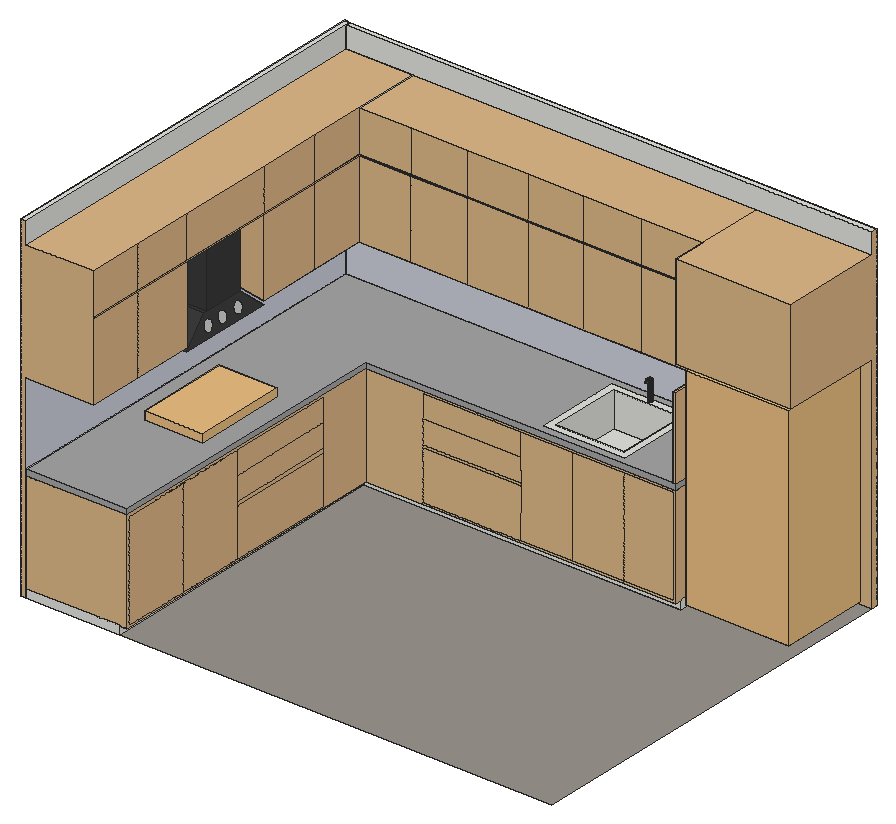
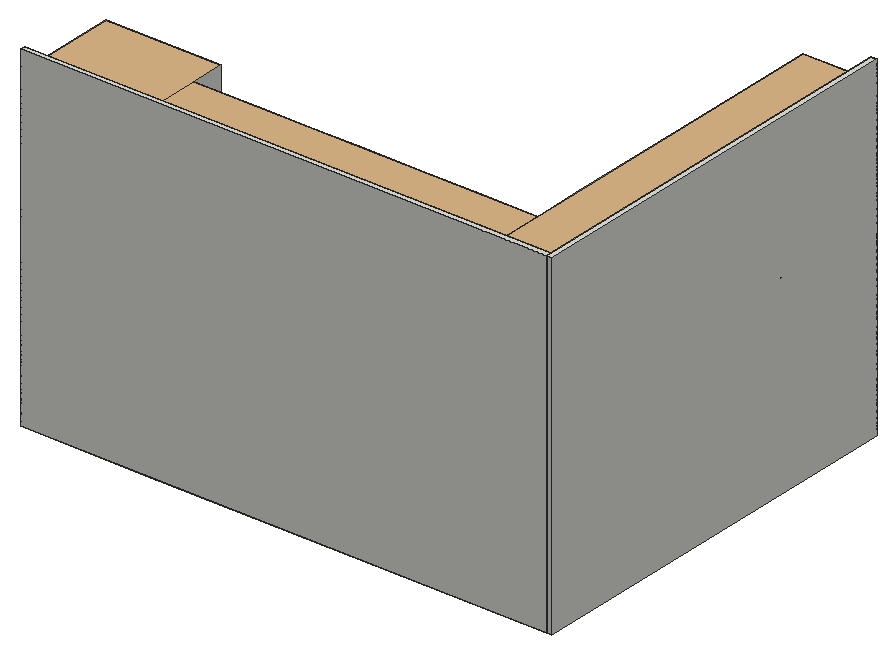
# SketchUp Ruby script. Lengths in inches.
U = 1.inch
M = Sketchup.active_model
def pt(a) = Geom::Point3d.new(a.map { |v| v * U })
def face(e, loops, mat)
  f = e.add_face(loops[0].map { |a| pt(a) })
  loops[1..].each { |l| e.add_face(l.map { |a| pt(a) }).erase! }
  f.material = f.back_material = mat if mat
  f
end
# faces: each face lists its corners as indices into pts; further lists are holes
def faces(e, pts, list, mat = nil) = list.each { |f| face(e, (f[0].is_a?(Array) ? f : [f]).map { |l| l.map { |i| pts[i] } }, mat) }
# xy, xz, yz: faces in a plane at the given z, y or x. An outline is a flat list of corners, or four numbers for a rectangle; further outlines are holes
def ring(l) = l.size == 4 ? [[l[0], l[1]], [l[2], l[1]], [l[2], l[3]], [l[0], l[3]]] : l.each_slice(2).to_a
def flat(e, list, mat, &to3) = list.each { |f| face(e, (f[0].is_a?(Array) ? f : [f]).map { |l| ring(l).map { |u, v| to3.(u, v) } }, mat) }
def xy(e, z, list, mat = nil) = flat(e, list, mat) { |x, y| [x, y, z] }
def xz(e, y, list, mat = nil) = flat(e, list, mat) { |x, z| [x, y, z] }
def yz(e, x, list, mat = nil) = flat(e, list, mat) { |y, z| [x, y, z] }
def lines(e, pts, list) = list.each { |a, b| e.add_line(pt(pts[a]), pt(pts[b])) }
# prism: a flat outline (further loops are holes) pulled along v
def prism(e, loops, v, mat = nil)
  f = face(e, loops, mat); d = Geom::Vector3d.new(v.map { |x| x * U })
  f.pushpull(f.normal.samedirection?(d) ? d.length : -d.length)
end
def box(e, o, s, mat = nil) = prism(e, [[o, [o[0] + s[0], o[1], o[2]], [o[0] + s[0], o[1] + s[1], o[2]], [o[0], o[1] + s[1], o[2]]]], [0, 0, s[2]], mat)
def at(x, y, z, deg = 0) = Geom::Transformation.translation(pt([x, y, z])) * Geom::Transformation.rotation(ORIGIN, Z_AXIS, deg.degrees)
def axes(o, x, y, z) = Geom::Transformation.new([*x, 0, *y, 0, *z, 0, *pt(o).to_a, 1])
def part(name) = M.definitions.add(name)
# library, detail: a bought-in or finely detailed component or shape, given as its bounding box
def library(name, o, s) = part(name).tap { |d| box(d.entities, o, s) }
def detail(e, o, s) = box(e.add_group.entities, o, s)
def put(e, d, t, mat = nil) = e.add_instance(d, t).tap { |i| i.material = mat if mat }
def group(e, t, mat = nil) = e.add_group.tap { |g| g.transformation = t; g.material = mat if mat }.entities
root = M.entities
M.materials.add("[0036_BurlyWood]").color = [222, 184, 135]
M.materials.add("[Color M02]").color = [198, 198, 198]
M.materials.add("[Color M06]").color = [86, 86, 86]
M.materials.add("[Color M07]").color = [58, 58, 58]
M.materials.add("[Granite Tile]").color = [155, 148, 143]
M.materials.add("[Marble Carrara Floor Tile]").color = [204, 208, 219]
M.materials.add("[Stone Vein Gray]").color = [166, 165, 165]
c1 = library("Group\#3",[0,0,0],[36.5,31.625,66.0625])
xy(root,0,[[0,0,2,144],[2,0,2,142,147.9375,142,147.9375,108.5,35.1875,108.5,35.1875,0],[2,142,147.9375,144],[147.9375,142,188.9375,144]])
xy(root,0,[[35.1875,0,35.1875,108.5,147.9375,108.5,147.9375,142,188.9375,142,188.9375,0]],"[Granite Tile]")
xy(root,3,[[2,0,2,142,147.9375,142,147.9375,108.5,35.1875,108.5,35.1875,0],[35.1875,0,38,108.5],[38,106,147.9375,108.5]])
xy(root,28,[[3.713,1.713,36.287,1.713,36.287,107.713,146.224,107.713,146.224,140.287,3.713,140.287]])
xy(root,28.6875,[[101.152,111.388,125.325,136.999]])
xy(root,39,[[[2,0,2,142,147.9375,142,147.9375,106,38,106,38,0],[3.713,1.713,36.287,1.713,36.287,107.713,146.224,107.713,146.224,140.287,3.713,140.287]]])
xy(root,41,[[[98.739,108.975,127.739,139.412],[101.152,111.388,125.325,136.999],[113.239,137.739,113.065,137.762,112.904,137.829,112.765,137.935,112.658,138.074,112.591,138.236,112.569,138.409,112.591,138.582,112.658,138.744,112.765,138.883,112.904,138.989,113.065,139.056,113.239,139.079,113.412,139.056,113.573,138.989,113.712,138.883,113.819,138.744,113.886,138.582,113.908,138.409,113.886,138.236,113.819,138.074,113.712,137.935,113.573,137.829,113.412,137.762]],[113.239,137.739,113.065,137.762,112.904,137.829,112.765,137.935,112.658,138.074,112.591,138.236,112.569,138.409,112.591,138.582,112.658,138.744,112.765,138.883,112.904,138.989,113.065,139.056,113.239,139.079,113.412,139.056,113.573,138.989,113.712,138.883,113.819,138.744,113.886,138.582,113.908,138.409,113.886,138.236,113.819,138.074,113.712,137.935,113.573,137.829,113.412,137.762]])
xy(root,41,[[146.9375,106,147.9375,142]],"[0036_BurlyWood]")
xy(root,41,[[[2,0,38,0,38,106,146.9375,106,146.9375,142,2,142],[98.739,108.975,127.739,139.412]]],"[Stone Vein Gray]")
xy(root,70,[[2,0,26,41.497],[26,75.622,2,79.962,2,142,26,142],[146.9375,106,147.9375,118],[26,118,146.9375,142],[146.9375,118,147.9375,142]],"[0036_BurlyWood]")
xy(root,79.249,[[147.9375,106,188.9375,142]],"[0036_BurlyWood]")
xy(root,97.4375,[[2,41.497,2,79.962,26,75.622,26,41.497]])
xy(root,97.613,[[125.9375,117.875,147.9375,118]],"[0036_BurlyWood]")
xy(root,97.614,[[26,0,26.3125,118],[26.3125,117.875,44.25,118],[44.25,117.875,64.75,118],[64.75,117.875,86,118],[86,117.875,105.3125,118],
  [105.3125,117.875,125.9375,118]],"[0036_BurlyWood]")
xy(root,97.929,[[26,0,26.3125,118],[26.3125,117.875,44.25,118],[44.25,117.875,64.75,118],[64.75,117.875,86,118],[86,117.875,105.3125,118],
  [105.3125,117.875,147.9375,118]],"[0036_BurlyWood]")
xy(root,112.601,[[2,0,26,142],[147.9375,106,188.9375,142],[26,118,147.9375,142]],"[0036_BurlyWood]")
xy(root,120,[[0,0,2,144],[2,142,188.9375,144]])
xz(root,0,[[2,0,35.1875,3]])
xz(root,0,[[0,0,2,0,2,70,26,70,26,97.614,26.3125,97.614,26.3125,97.929,26,97.929,26,112.601,2,112.601,2,120,0,120],[2,3,38,39]],"[0036_BurlyWood]")
xz(root,0,[[2,39,38,41]],"[Stone Vein Gray]")
xz(root,1.713,[[3.713,28,36.287,39]])
xz(root,41.497,[[2,70,26,97.4375]],"[0036_BurlyWood]")
xz(root,106,[[[38,3,147.9375,39],[58.162,3.56,58.287,21,58.287,21.974,58.224,30.207,58.162,38.44,147.378,38.44,147.378,3.56]],[58.162,3.56,92.787,3.56,92.912,21,58.287,21],[92.787,3.56,111.037,3.56,111.037,38.44,92.787,38.44,92.849,30.207,92.912,21.974,92.912,21],[111.037,3.56,129.537,38.44],[129.537,3.56,147.378,38.44],
  [58.287,21,92.912,21.974],[58.287,21.974,92.912,21.974,92.849,30.207,58.224,30.207],[58.224,30.207,92.849,30.207,92.787,38.44,58.162,38.44],[146.9375,41,147.9375,70],[147.9375,79.249,188.9375,112.601]],"[0036_BurlyWood]")
xz(root,106,[[38,39,147.9375,41]],"[Stone Vein Gray]")
xz(root,107.713,[[36.287,28,146.224,39]])
xz(root,108.5,[[35.1875,0,147.9375,3]])
xz(root,111.388,[[101.152,28.6875,125.325,41]])
xz(root,117.875,[[125.9375,97.613,147.9375,97.613,147.9375,97.929,105.3125,97.929,105.3125,97.614,125.9375,97.614],[26.3125,97.614,44.25,97.929],[44.25,97.614,64.75,97.929],[64.75,97.614,86,97.929],[86,97.614,105.3125,97.929]],"[0036_BurlyWood]")
xz(root,118,[[26,97.614,26.3125,97.8],[26,97.8,26.3125,97.929]])
xz(root,118,[[26,70,44.25,97.614],[44.25,70,64.75,97.614],[64.75,70,86,97.614],[86,70,105.3125,97.614],[105.3125,70,125.9375,97.614],
  [125.9375,70,147.9375,97.613],[26,97.929,44.25,112.601],[44.25,97.929,64.75,112.601],[64.75,97.929,86,112.601],[86,97.929,105.3125,112.601],
  [105.3125,97.929,125.9375,112.601],[125.9375,97.929,147.9375,112.601]],"[0036_BurlyWood]")
xz(root,136.999,[[101.152,28.6875,125.325,41]])
xz(root,140.287,[[3.713,28,146.224,39]])
xz(root,142,[[2,0,147.9375,3],[2,3,147.9375,39],[2,39,147.9375,41],[2,70,26,112.601],[2,112.601,188.9375,120]])
xz(root,142,[[147.9375,0,188.9375,79.249],[146.9375,41,147.9375,70]],"[0036_BurlyWood]")
xz(root,142,[[2,41,146.9375,70]],"[Marble Carrara Floor Tile]")
xz(root,144,[[0,0,2,120],[2,0,188.9375,120]])
yz(root,0,[[0,0,144,120]])
yz(root,2,[[0,0,142,3],[142,0,144,120],[0,3,142,39],[0,39,142,41],[0,112.601,142,120]])
yz(root,2,[[0,41,142,41,142,70,79.962,70,79.962,97.4375,41.497,97.4375,41.497,70,0,70]],"[Marble Carrara Floor Tile]")
yz(root,3.713,[[1.713,28,140.287,39]])
yz(root,26,[[118,70,142,112.601],[41.497,97.4375,75.622,97.614]])
yz(root,26,[[0,70,19.625,97.614],[19.625,70,41.497,97.614],[75.622,70,98.247,97.614],[98.247,70,118,97.614],[0,97.929,19.625,112.601],
  [19.625,97.929,41.497,112.601],[41.497,97.929,75.622,112.601],[75.622,97.929,98.247,112.601],[98.247,97.929,118,112.601]],"[0036_BurlyWood]")
yz(root,26.3125,[[117.875,97.614,118,97.929]])
yz(root,26.3125,[[0,97.614,117.875,97.929]],"[0036_BurlyWood]")
yz(root,35.1875,[[0,0,108.5,3]])
yz(root,36.287,[[1.713,28,107.713,39]])
yz(root,38,[[[0,3,106,39],[0.581,3.581,0.581,38.419,86.83,38.419,86.865,30.341,86.901,21.937,86.901,20.438,86.83,3.581]],[0.581,3.581,24.517,38.419],[24.517,3.581,48.892,3.581,48.963,20.438,48.963,21.937,48.928,30.178,48.892,38.419,24.517,38.419],[48.892,3.581,86.83,3.581,86.901,20.438,48.963,20.438],[48.963,20.438,86.901,21.937],
  [48.963,21.937,86.901,21.937,86.865,30.341,48.928,30.178],[48.928,30.178,86.865,30.341,86.83,38.419,48.892,38.419]],"[0036_BurlyWood]")
yz(root,38,[[0,39,106,41]],"[Stone Vein Gray]")
yz(root,101.152,[[111.388,28.6875,136.999,41]])
yz(root,125.325,[[111.388,28.6875,136.999,38.375],[111.388,38.375,136.999,41]])
yz(root,125.9375,[[117.875,97.613,118,97.614]])
yz(root,146.224,[[107.713,28,140.287,39]])
yz(root,146.9375,[[106,41,142,70]],"[0036_BurlyWood]")
yz(root,147.9375,[[108.5,0,142,3],[106,79.249,106,112.601,118,112.601,118,97.929,117.875,97.929,117.875,97.613,118,97.613,118,79.249]])
yz(root,147.9375,[[106,3,142,39],[106,41,142,70],[118,70,142,79.249]],"[0036_BurlyWood]")
yz(root,147.9375,[[106,39,142,41]],"[Stone Vein Gray]")
yz(root,188.9375,[[142,0,144,0,144,120,142,120,142,112.601,106,112.601,106,79.249,142,79.249]],"[0036_BurlyWood]")
p = [[113.065,137.762,41],[113.239,137.739,41],[113.239,137.739,47.367],[113.239,137.739,47.377],[113.065,137.762,47.381],[113.065,137.762,47.373],
  [113.412,137.762,41],[113.412,137.762,47.373],[113.412,137.762,47.381],[112.765,137.935,41],[112.904,137.829,41],[112.904,137.829,47.394],
  [112.901,137.83,47.394],[112.765,137.935,47.413],[113.573,137.829,41],[113.573,137.829,47.394],[113.712,137.935,41],[113.712,137.935,47.413],
  [113.576,137.83,47.394],[112.658,138.074,41],[112.658,138.074,47.439],[113.819,138.074,41],[113.819,138.074,47.439],[112.591,138.236,41],
  [112.591,138.236,47.468],[113.886,138.236,41],[113.886,138.236,47.468],[112.569,138.409,41],[112.569,138.409,47.5],[113.908,138.409,41],
  [113.908,138.409,47.5],[112.591,138.582,41],[112.591,138.582,47.532],[113.886,138.582,41],[113.886,138.582,47.532],[112.658,138.744,41],
  [112.658,138.744,47.561],[113.819,138.744,41],[113.819,138.744,47.561],[112.765,138.883,41],[112.765,138.883,47.587],[113.712,138.883,41],
  [113.712,138.883,47.587],[112.904,138.989,41],[112.904,138.989,47.606],[113.573,138.989,41],[113.573,138.989,47.606],[113.065,139.056,41],
  [113.065,139.056,47.619],[113.412,139.056,41],[113.412,139.056,47.619],[113.239,139.079,41],[113.239,139.079,47.623],[112.569,136.909,47.5],
  [112.591,137.071,47.439],[112.658,137.222,47.381],[112.765,137.352,47.332],[112.904,137.451,47.294],[113.065,137.514,47.271],[113.239,137.535,47.262],
  [113.412,137.514,47.271],[113.573,137.451,47.294],[113.712,137.352,47.332],[113.819,137.222,47.381],[113.886,137.071,47.439],[113.908,136.909,47.5],
  [113.886,136.747,47.561],[113.819,136.596,47.619],[113.712,136.466,47.668],[113.573,136.366,47.706],[113.412,136.304,47.729],[113.239,136.283,47.738],
  [113.065,136.304,47.729],[112.904,136.366,47.706],[112.765,136.466,47.668],[112.658,136.596,47.619],[112.591,136.747,47.561],[112.658,137.269,47.505],
  [112.765,137.394,47.442],[113.712,137.394,47.442],[113.819,137.269,47.505],[112.904,137.489,47.393],[113.573,137.489,47.393],[113.065,137.549,47.363],
  [113.239,137.569,47.352],[113.412,137.549,47.363],[112.569,136.969,47.659],[112.591,137.125,47.579],[113.886,137.125,47.579],[113.908,136.969,47.659],
  [112.658,137.322,47.586],[112.765,137.429,47.497],[113.712,137.429,47.497],[113.819,137.322,47.586],[112.904,137.512,47.428],[112.765,137.476,47.542],
  [112.904,137.542,47.457],[113.573,137.542,47.457],[113.712,137.476,47.542],[113.573,137.512,47.428],[112.904,137.578,47.479],[113.065,137.606,47.418],
  [113.065,137.583,47.404],[113.065,137.564,47.385],[113.239,137.581,47.371],[113.412,137.564,47.385],[113.412,137.606,47.418],[113.573,137.578,47.479],
  [113.412,137.583,47.404],[112.904,137.659,47.497],[113.065,137.659,47.43],[113.065,137.632,47.427],[112.904,137.617,47.493],[113.239,137.659,47.407],
  [113.239,137.637,47.405],[113.239,137.616,47.397],[113.239,137.597,47.386],[113.412,137.659,47.43],[113.412,137.632,47.427],[113.573,137.659,47.497],
  [113.573,137.617,47.493],[112.904,137.806,47.428],[113.065,137.754,47.385],[113.065,137.735,47.404],[112.904,137.776,47.457],[113.065,137.712,47.418],
  [112.904,137.74,47.479],[113.065,137.686,47.427],[112.904,137.701,47.493],[113.065,137.769,47.363],[113.239,137.749,47.352],[113.239,137.736,47.371],
  [113.239,137.721,47.386],[113.239,137.702,47.397],[113.239,137.681,47.405],[113.412,137.769,47.363],[113.412,137.754,47.385],[113.412,137.735,47.404],
  [113.412,137.712,47.418],[113.412,137.686,47.427],[113.573,137.806,47.428],[113.573,137.776,47.457],[113.573,137.74,47.479],[113.573,137.701,47.493],
  [112.765,137.924,47.442],[112.765,137.888,47.497],[112.765,137.841,47.542],[113.712,137.924,47.442],[113.712,137.888,47.497],[113.712,137.841,47.542],
  [112.658,138.049,47.505],[112.658,137.996,47.586],[113.819,138.049,47.505],[113.819,137.996,47.586],[112.591,138.193,47.579],[113.886,138.193,47.579],
  [112.591,136.814,47.738],[113.886,136.814,47.738],[112.591,137.197,47.689],[113.886,137.197,47.689],[112.658,137.391,47.652],[113.819,137.391,47.652],
  [112.658,137.473,47.702],[112.765,137.532,47.576],[113.712,137.532,47.576],[113.819,137.473,47.702],[112.765,137.594,47.597],[113.712,137.594,47.597],
  [112.765,137.659,47.604],[113.712,137.659,47.604],[112.765,137.786,47.576],[112.765,137.724,47.597],[113.712,137.786,47.576],[113.712,137.724,47.597],
  [112.658,137.927,47.652],[112.658,137.845,47.702],[113.819,137.927,47.652],[113.819,137.845,47.702],[112.591,138.121,47.689],[113.886,138.121,47.689],
  [112.569,138.349,47.659],[113.908,138.349,47.659],[112.591,138.504,47.738],[113.886,138.504,47.738],[112.658,138.649,47.812],[113.819,138.649,47.812],
  [112.765,136.545,47.876],[112.658,136.669,47.812],[113.819,136.669,47.812],[113.712,136.545,47.876],[112.569,137.0625,47.801],[113.908,137.0625,47.801],
  [112.591,137.291,47.781],[113.886,137.291,47.781],[112.658,137.564,47.733],[113.819,137.564,47.733],[112.658,137.659,47.744],[113.819,137.659,47.744],
  [112.658,137.754,47.733],[113.819,137.754,47.733],[112.591,138.026,47.781],[113.886,138.026,47.781],[112.569,138.255,47.801],[113.908,138.255,47.801],
  [112.765,138.773,47.876],[113.712,138.773,47.876],[112.904,138.869,47.924],[113.573,138.869,47.924],[113.065,138.928,47.955],[113.239,138.949,47.965],
  [113.412,138.928,47.955],[113.065,136.389,47.955],[112.904,136.449,47.924],[113.239,136.369,47.965],[113.412,136.389,47.955],[113.573,136.449,47.924],
  [112.658,136.803,48.016],[112.591,136.928,47.912],[113.886,136.928,47.912],[113.819,136.803,48.016],[112.569,137.185,47.919],[113.908,137.185,47.919],
  [112.591,137.404,47.85],[113.886,137.404,47.85],[112.591,137.528,47.892],[113.886,137.528,47.892],[112.591,137.659,47.907],[113.886,137.659,47.907],
  [112.591,137.79,47.892],[113.886,137.79,47.892],[112.591,137.914,47.85],[113.886,137.914,47.85],[112.569,138.133,47.919],[113.908,138.133,47.919],
  [112.591,138.39,47.912],[113.886,138.39,47.912],[112.658,138.515,48.016],[113.819,138.515,48.016],[112.765,136.696,48.105],[113.712,136.696,48.105],
  [112.591,137.078,48.057],[113.886,137.078,48.057],[112.569,137.329,48.007],[113.908,137.329,48.007],[112.569,137.49,48.0625],[113.908,137.49,48.0625],
  [112.569,137.988,48.007],[112.569,137.828,48.0625],[113.908,137.988,48.007],[113.908,137.828,48.0625],[112.591,138.24,48.057],[113.886,138.24,48.057],
  [112.765,138.622,48.105],[113.712,138.622,48.105],[112.904,136.613,48.173],[113.065,136.561,48.216],[113.573,136.613,48.173],[113.412,136.561,48.216],
  [112.658,136.978,48.185],[113.819,136.978,48.185],[112.591,137.255,48.165],[113.886,137.255,48.165],[112.569,137.659,48.081],[113.908,137.659,48.081],
  [112.591,138.0625,48.165],[113.886,138.0625,48.165],[112.658,138.34,48.185],[113.819,138.34,48.185],[112.904,138.705,48.173],[113.573,138.705,48.173],
  [113.065,138.757,48.216],[113.412,138.757,48.216],[113.239,136.544,48.231],[112.765,136.893,48.296],[113.712,136.893,48.296],[112.591,137.452,48.233],
  [113.886,137.452,48.233],[112.591,137.866,48.233],[113.886,137.866,48.233],[112.765,138.425,48.296],[113.712,138.425,48.296],[113.239,138.774,48.231],
  [112.904,136.827,48.38],[113.573,136.827,48.38],[112.658,137.186,48.3125],[113.819,137.186,48.3125],[112.591,137.659,48.255],[113.886,137.659,48.255],
  [112.658,138.132,48.3125],[113.819,138.132,48.3125],[112.904,138.491,48.38],[113.573,138.491,48.38],[113.239,136.772,48.452],[113.065,136.786,48.433],
  [113.412,136.786,48.433],[112.765,137.127,48.439],[113.712,137.127,48.439],[112.658,137.417,48.391],[113.819,137.417,48.391],[112.658,137.659,48.418],
  [113.819,137.659,48.418],[112.658,137.901,48.391],[113.819,137.901,48.391],[112.765,138.191,48.439],[113.712,138.191,48.439],[113.065,138.532,48.433],
  [113.239,138.546,48.452],[113.412,138.532,48.433],[112.904,137.081,48.536],[113.573,137.081,48.536],[112.765,137.386,48.527],[113.712,137.386,48.527],
  [112.765,137.932,48.527],[113.712,137.932,48.527],[112.904,138.237,48.536],[113.573,138.237,48.536],[113.065,137.053,48.597],[113.239,137.043,48.617],
  [113.412,137.053,48.597],[112.904,137.363,48.632],[113.573,137.363,48.632],[112.765,137.659,48.558],[113.712,137.659,48.558],[112.904,137.955,48.632],
  [113.573,137.955,48.632],[113.065,138.265,48.597],[113.412,138.265,48.597],[113.239,138.275,48.617],[113.065,137.348,48.698],[113.412,137.348,48.698],
  [112.904,137.659,48.665],[113.573,137.659,48.665],[113.065,137.97,48.698],[113.412,137.97,48.698],[113.239,137.343,48.72],[113.065,137.659,48.732],
  [113.412,137.659,48.732],[113.239,137.975,48.72],[113.239,137.659,48.755],[2,79.962,70],[26,75.622,70],[26,75.622,97.4375],
  [2,79.962,97.4375],[113.239,138.409,41],[113.239,138.409,47.5],[113.239,138.349,47.659],[113.239,138.255,47.801],[113.239,138.133,47.919],
  [113.239,137.988,48.007],[113.239,137.828,48.0625],[113.239,137.659,48.081],[113.239,137.49,48.0625],[113.239,137.329,48.007],[113.239,137.185,47.919],
  [113.239,137.0625,47.801],[113.239,136.969,47.659],[113.239,136.909,47.5],[146.224,140.287,39],[146.224,140.287,41],[3.713,140.287,39],
  [3.713,140.287,41],[36.287,1.713,39],[36.287,1.713,41],[36.287,107.713,39],[36.287,107.713,41],[146.224,107.713,39],
  [146.224,107.713,41],[3.713,1.713,39],[3.713,1.713,41]]
faces(root,p,[[0,1,2,3,4,5],[1,6,7,8,3,2],[9,10,11,12,13],[10,0,5,4,11],[6,14,15,8,7],[14,16,17,18,15],[19,9,13,20],[16,21,22,17],
  [23,19,20,24],[21,25,26,22],[27,23,24,28],[25,29,30,26],[31,27,28,32],[29,33,34,30],[35,31,32,36],[33,37,38,34],
  [39,35,36,40],[37,41,42,38],[43,39,40,44],[41,45,46,42],[47,43,44,48],[45,49,50,46],[51,47,48,52],[49,51,52,50],
  [77,78,56,55],[79,80,63,62],[78,81,57,56],[82,79,62,61],[81,83,58,57],[83,84,59,58],[84,85,60,59],[85,82,61,60],
  [86,87,54,53],[88,89,65,64],[87,77,55,54],[80,88,64,63],[90,91,78,77],[92,93,80,79],[91,94,81,78],[95,96,94,91],
  [97,98,92,99],[99,92,79,82],[100,101,102,96],[96,102,103,94],[94,103,83,81],[103,104,84,83],[104,105,85,84],[106,107,97,108],
  [108,97,99,105],[105,99,82,85],[109,110,111,112],[112,111,101,100],[110,113,114,111],[111,114,115,101],[101,115,116,102],[102,116,104,103],
  [113,117,118,114],[114,118,106,115],[115,106,108,116],[116,108,105,104],[117,119,120,118],[118,120,107,106],[121,122,123,124],[124,123,125,126],
  [126,125,127,128],[128,127,110,109],[129,130,2,131,122,5],[122,131,132,123],[123,132,133,125],[125,133,134,127],[127,134,113,110],[130,135,7,136,131,2],
  [131,136,137,132],[132,137,138,133],[133,138,139,134],[134,139,117,113],[136,140,141,137],[137,141,142,138],[138,142,143,139],[139,143,119,117],
  [144,12,11,121,145],[144,13,12],[145,121,124,146],[11,129,5,122,121],[135,15,140,136,7],[15,18,147,148,140],[17,147,18],[140,148,149,141],
  [150,144,145,151],[20,13,144,150],[147,152,153,148],[17,22,152,147],[24,20,150,154],[22,26,155,152],[156,86,53,76],[89,157,66,65],
  [158,90,77,87],[93,159,88,80],[160,95,91,90],[98,161,93,92],[162,163,95,160],[164,165,161,98],[166,112,100,163],[163,100,96,95],
  [120,167,164,107],[107,164,98,97],[168,109,112,166],[119,169,167,120],[146,124,126,170],[170,126,128,171],[171,128,109,168],[141,149,172,142],
  [142,172,173,143],[143,173,169,119],[151,145,146,174],[174,146,170,175],[148,153,176,149],[149,176,177,172],[154,150,151,178],[152,155,179,153],
  [28,24,154,180],[26,30,181,155],[32,28,180,182],[30,34,183,181],[36,32,182,184],[34,38,185,183],[186,187,75,74],[188,189,68,67],
  [187,156,76,75],[157,188,67,66],[190,158,87,86],[159,191,89,88],[192,160,90,158],[161,193,159,93],[194,166,163,162],[167,195,165,164],
  [196,168,166,194],[169,197,195,167],[175,170,171,198],[198,171,168,196],[172,177,199,173],[173,199,197,169],[178,151,174,200],[153,179,201,176],
  [180,154,178,202],[155,181,203,179],[40,36,184,204],[38,42,205,185],[44,40,204,206],[42,46,207,205],[48,44,206,208],[52,48,208,209],
  [50,52,209,210],[46,50,210,207],[211,212,73,72],[213,211,72,71],[214,213,71,70],[215,214,70,69],[212,186,74,73],[189,215,69,68],
  [216,217,156,187],[218,219,188,157],[217,190,86,156],[191,218,157,89],[220,192,158,190],[193,221,191,159],[222,162,160,192],[165,223,193,161],
  [224,194,162,222],[195,225,223,165],[226,196,194,224],[197,227,225,195],[228,198,196,226],[199,229,227,197],[200,174,175,230],[230,175,198,228],
  [176,201,231,177],[177,231,229,199],[202,178,200,232],[179,203,233,201],[182,180,202,234],[181,183,235,203],[184,182,234,236],[183,185,237,235],
  [238,216,187,186],[219,239,189,188],[240,220,190,217],[221,241,218,191],[242,222,192,220],[223,243,221,193],[244,224,222,242],[225,245,243,223],
  [246,230,228,247],[231,248,249,229],[232,200,230,246],[201,233,248,231],[234,202,232,250],[203,235,251,233],[204,184,236,252],[185,205,253,237],
  [254,238,186,212],[255,254,212,211],[256,257,214,215],[239,256,215,189],[258,240,217,216],[241,259,219,218],[260,242,220,240],[243,261,241,221],
  [262,226,224,244],[227,263,245,225],[247,228,226,262],[229,249,263,227],[250,232,246,264],[233,251,265,248],[236,234,250,266],[235,237,267,251],
  [206,204,252,268],[205,207,269,253],[208,206,268,270],[207,210,271,269],[272,255,211,213],[257,272,213,214],[273,258,216,238],[259,274,239,219],
  [275,244,242,260],[245,276,261,243],[264,246,247,277],[248,265,278,249],[252,236,266,279],[237,253,280,267],[209,208,270,281],[210,209,281,271],
  [282,273,238,254],[274,283,256,239],[284,260,240,258],[261,285,259,241],[286,262,244,275],[263,287,276,245],[277,247,262,286],[249,278,287,263],
  [266,250,264,288],[251,267,289,265],[268,252,279,290],[253,269,291,280],[292,293,255,272],[294,292,272,257],[293,282,254,255],[283,294,257,256],
  [295,284,258,273],[285,296,274,259],[297,275,260,284],[276,298,285,261],[299,286,275,297],[287,300,298,276],[301,277,286,299],[278,302,300,287],
  [288,264,277,301],[265,289,302,278],[279,266,288,303],[267,280,304,289],[270,268,290,305],[281,270,305,306],[271,281,306,307],[269,271,307,291],
  [308,295,273,282],[296,309,283,274],[310,297,284,295],[298,311,296,285],[303,288,301,312],[289,304,313,302],[290,279,303,314],[280,291,315,304],
  [316,308,282,293],[317,316,293,292],[318,317,292,294],[309,318,294,283],[319,310,295,308],[311,320,309,296],[321,299,297,310],[300,322,311,298],
  [312,301,299,321],[302,313,322,300],[314,303,312,323],[304,315,324,313],[305,290,314,325],[291,307,326,315],[306,305,325,327],[307,306,327,326],
  [328,319,308,316],[320,329,318,309],[330,321,310,319],[322,331,320,311],[323,312,321,330],[313,324,331,322],[325,314,323,332],[315,326,333,324],
  [334,328,316,317],[329,334,317,318],[335,330,319,328],[331,336,329,320],[332,323,330,335],[324,333,336,331],[327,325,332,337],[326,327,337,333],
  [338,335,328,334],[336,338,334,329],[337,332,335,338],[333,337,338,336]],"[Color M06]")
faces(root,p,[[53,54,55,56,57,58,59,60,61,62,63,64,65,66,67,68,69,70,71,72,73,74,75,76]])
faces(root,p,[[339,340,341,342]],"[0036_BurlyWood]")
lines(root,p,[[343,344],[344,345],[345,346],[346,347],[347,348],[348,349],[349,350],[350,351],[351,352],[352,353],[353,354],[354,355],
  [355,356],[357,358],[359,360],[361,362],[363,364],[365,366],[367,368]])
detail(root,[10.29,42.33,41],[20.62,33.06,3])
g1 = group(root,at(9.91,53.1,75.72))
box(g1,[0,0,0],[13.82,14.875,21.72],"[Color M07]")
g2 = group(root,at(0,41.5,68.52))
xy(g2,0,[[[0,0,26,34.125],[1.92,1.52,24.08,32.61]],[1.92,1.52,24.08,32.61]],"[Color M07]")
xy(g2,7.2,[[9.61,10.1875,23.74,26.48]],"[Color M07]")
p = [[0,0,0],[9.61,10.1875,7.2],[9.61,26.48,7.2],[0,34.125,0],[26,0,0],[23.74,10.1875,7.2],
  [26,34.125,0],[23.74,26.48,7.2],[24.33,10.94,5.32],[24.36,11.42,5.21],[24.4375,11.87,4.97],[24.55,12.23,4.62],
  [24.68,12.5,4.18],[24.84,12.64,3.69],[25,12.66,3.18],[25.16,12.55,2.68],[25.3,12.3125,2.23],[25.42,11.97,1.86],
  [25.5,11.54,1.59],[25.55,11.0625,1.44],[25.55,10.5625,1.42],[25.52,10.07,1.54],[25.44,9.63,1.78],[25.33,9.26,2.13],
  [25.19,9,2.5625],[25.04,8.85,3.05],[24.88,8.84,3.5625],[24.72,8.95,4.06],[24.58,9.1875,4.51],[24.46,9.53,4.89],
  [24.38,9.95,5.16],[24.33,10.43,5.3],[24.84,18.94,3.69],[25,18.96,3.18],[25.16,18.85,2.68],[25.3,18.61,2.23],
  [25.42,18.27,1.86],[25.5,17.84,1.59],[25.55,17.36,1.44],[25.55,16.86,1.42],[25.52,16.37,1.54],[25.44,15.93,1.78],
  [25.33,15.5625,2.13],[25.19,15.3,2.5625],[25.04,15.15,3.05],[24.88,15.13,3.5625],[24.72,15.25,4.06],[24.58,15.48,4.51],
  [24.46,15.83,4.89],[24.38,16.25,5.16],[24.33,16.73,5.3],[24.33,17.23,5.32],[24.36,17.72,5.21],[24.4375,18.17,4.97],
  [24.55,18.53,4.62],[24.68,18.8,4.18],[24.84,25.88,3.69],[25,25.9,3.18],[25.16,25.79,2.68],[25.3,25.55,2.23],
  [25.42,25.21,1.86],[25.5,24.78,1.59],[25.55,24.3,1.44],[25.55,23.8,1.42],[25.52,23.3125,1.54],[25.44,22.87,1.78],
  [25.33,22.5,2.13],[25.19,22.24,2.5625],[25.04,22.09,3.05],[24.88,22.07,3.5625],[24.72,22.1875,4.06],[24.58,22.42,4.51],
  [24.46,22.77,4.89],[24.38,23.19,5.16],[24.33,23.67,5.3],[24.33,24.17,5.32],[24.36,24.66,5.21],[24.4375,25.1,4.97],
  [24.55,25.47,4.62],[24.68,25.74,4.18]]
faces(g2,p,[[0,1,2,3],[0,4,5,1],[[4,6,7,5],[8,9,10,11,12,13,14,15,16,17,18,19,20,21,22,23,24,25,26,27,28,29,30,31],[32,33,34,35,36,37,38,39,40,41,42,43,44,45,46,47,48,49,50,51,52,53,54,55],[56,57,58,59,60,61,62,63,64,65,66,67,68,69,70,71,72,73,74,75,76,77,78,79]],[3,2,7,6]],"[Color M07]")
faces(g2,p,[[9,8,31,30,29,28,27,26,25,24,23,22,21,20,19,18,17,16,15,14,13,12,11,10],[52,51,50,49,48,47,46,45,44,43,42,41,40,39,38,37,36,35,34,33,32,55,54,53],[76,75,74,73,72,71,70,69,68,67,66,65,64,63,62,61,60,59,58,57,56,79,78,77]],"[Color M02]")
put(root,c1,axes([151.28,106.4,3.5],[1,0,0],[0,1,0],[0,0,1.13]))
